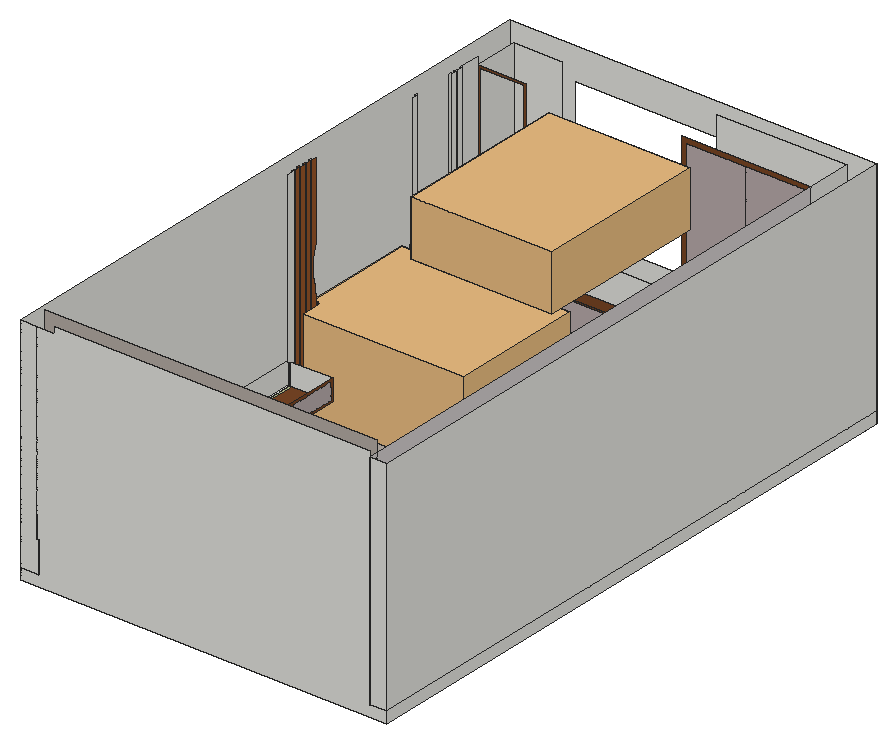
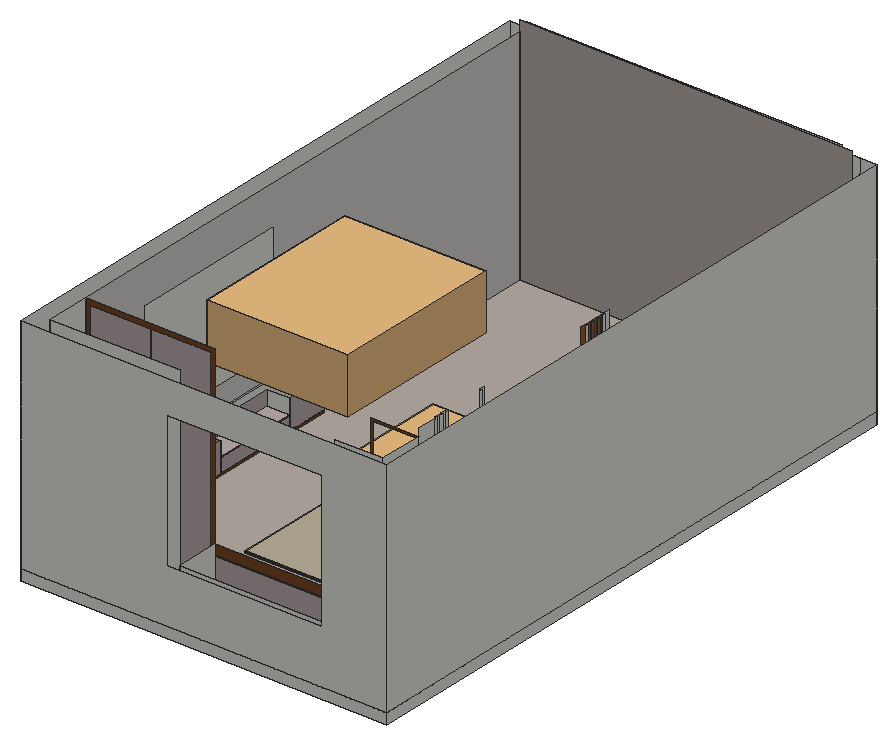
# SketchUp Ruby script. Lengths in inches.
U = 1.inch
M = Sketchup.active_model
def pt(a) = Geom::Point3d.new(a.map { |v| v * U })
def face(e, loops, mat)
  f = e.add_face(loops[0].map { |a| pt(a) })
  loops[1..].each { |l| e.add_face(l.map { |a| pt(a) }).erase! }
  f.material = f.back_material = mat if mat
  f
end
# faces: each face lists its corners as indices into pts; further lists are holes
def faces(e, pts, list, mat = nil) = list.each { |f| face(e, (f[0].is_a?(Array) ? f : [f]).map { |l| l.map { |i| pts[i] } }, mat) }
# xy, xz, yz: faces in a plane at the given z, y or x. An outline is a flat list of corners, or four numbers for a rectangle; further outlines are holes
def ring(l) = l.size == 4 ? [[l[0], l[1]], [l[2], l[1]], [l[2], l[3]], [l[0], l[3]]] : l.each_slice(2).to_a
def flat(e, list, mat, &to3) = list.each { |f| face(e, (f[0].is_a?(Array) ? f : [f]).map { |l| ring(l).map { |u, v| to3.(u, v) } }, mat) }
def xy(e, z, list, mat = nil) = flat(e, list, mat) { |x, y| [x, y, z] }
def xz(e, y, list, mat = nil) = flat(e, list, mat) { |x, z| [x, y, z] }
def yz(e, x, list, mat = nil) = flat(e, list, mat) { |y, z| [x, y, z] }
def lines(e, pts, list) = list.each { |a, b| e.add_line(pt(pts[a]), pt(pts[b])) }
# prism: a flat outline (further loops are holes) pulled along v
def prism(e, loops, v, mat = nil)
  f = face(e, loops, mat); d = Geom::Vector3d.new(v.map { |x| x * U })
  f.pushpull(f.normal.samedirection?(d) ? d.length : -d.length)
end
def box(e, o, s, mat = nil) = prism(e, [[o, [o[0] + s[0], o[1], o[2]], [o[0] + s[0], o[1] + s[1], o[2]], [o[0], o[1] + s[1], o[2]]]], [0, 0, s[2]], mat)
def at(x, y, z, deg = 0) = Geom::Transformation.translation(pt([x, y, z])) * Geom::Transformation.rotation(ORIGIN, Z_AXIS, deg.degrees)
def axes(o, x, y, z) = Geom::Transformation.new([*x, 0, *y, 0, *z, 0, *pt(o).to_a, 1])
def part(name) = M.definitions.add(name)
# library, detail: a bought-in or finely detailed component or shape, given as its bounding box
def library(name, o, s) = part(name).tap { |d| box(d.entities, o, s) }
def detail(e, o, s) = box(e.add_group.entities, o, s)
def put(e, d, t, mat = nil) = e.add_instance(d, t).tap { |i| i.material = mat if mat }
def group(e, t, mat = nil) = e.add_group.tap { |g| g.transformation = t; g.material = mat if mat }.entities
root = M.entities
M.materials.add("Ashlee 5_ x 8_").color = [182, 173, 150]
M.materials.add("Emissive").color = [188, 193, 143]
M.materials.add("Generic").color = [183, 170, 170]
M.materials.add("Generic\#1").color = [209, 204, 204]
M.materials.add("Tiles L01 200cm").color = [180, 171, 163]
M.materials.add("[Wood Cherry Original]").color = [152, 86, 42]
M.materials.add("[Wood Veneer 01]").color = [120, 70, 37]
c1 = library("ceiling fan",[0,0,0],[76.25,93.13,30.02])
c2 = part("fan")
p = [[217.527,-902.72,540.318],[217.529,-902.72,540.318],[217.529,-902.72,541.354],[217.527,-902.72,541.354]]
lines(c2.entities,p,[[0,1],[2,3]])
put(c2.entities,c1,at(256.45,-350.9,679.41))
c3 = library("BED 3",[-244.73,-59.6875,196.6875],[91.01,69.4,39.64])
c4 = part(" rug 5'x8'\#1")
xy(c4.entities,0,[[0,0,60,96]],"Ashlee 5_ x 8_")
xy(c4.entities,0.75,[[0.25,0.25,59.75,95.75]],"Ashlee 5_ x 8_")
xz(c4.entities,0,[[0,0,60,0.5]],"Ashlee 5_ x 8_")
xz(c4.entities,96,[[0,0,60,0.5]],"Ashlee 5_ x 8_")
yz(c4.entities,0,[[0,0,96,0.5]],"Ashlee 5_ x 8_")
yz(c4.entities,60,[[0,0,96,0.5]],"Ashlee 5_ x 8_")
p = [[59.99,0.01,0.56],[0.01,0.01,0.56],[0,0,0.5],[60,0,0.5],[0.01,95.99,0.56],[0,96,0.5],
  [59.99,95.99,0.56],[60,96,0.5],[0.03,0.03,0.625],[0.03,95.97,0.625],[59.97,0.03,0.625],[59.93,0.07,0.68],
  [0.07,0.07,0.68],[0.07,95.93,0.68],[59.93,95.93,0.68],[59.97,95.97,0.625],[0.125,0.125,0.72],[0.125,95.875,0.72],
  [59.81,0.19,0.74],[0.19,0.19,0.74],[59.875,0.125,0.72],[0.19,95.81,0.74],[59.81,95.81,0.74],[59.875,95.875,0.72],
  [0.25,0.25,0.75],[0.25,95.75,0.75],[59.75,0.25,0.75],[59.75,95.75,0.75]]
faces(c4.entities,p,[[0,1,2,3],[1,4,5,2],[6,0,3,7],[4,6,7,5],[8,9,4,1],[10,8,1,0],[11,12,8,10],[12,13,9,8],
  [14,11,10,15],[15,10,0,6],[13,14,15,9],[9,15,6,4],[16,17,13,12],[18,19,16,20],[20,16,12,11],[19,21,17,16],
  [22,18,20,23],[23,20,11,14],[24,25,21,19],[26,24,19,18],[27,26,18,22],[21,22,23,17],[25,27,22,21],[17,23,14,13]],"Ashlee 5_ x 8_")
xy(root,-6,[[0,0,198,331.1875]])
xy(root,0,[[0,0,9.9375,0,9.9375,172.18,9,172.18,9,173.55,9.9375,173.55,9.9375,175.97,9,175.97,9,177.34,9.9375,177.34,9.9375,179.77,9,179.77,9,181.13,9.9375,181.13,9.9375,183.56,9,183.56,9,184.92,9.9375,184.92,9.9375,187.35,9,187.35,9,188.71,9.8125,188.71,9.8125,191.14,9,191.14,9,192.51,9.8125,192.51,9.8125,194.93,9,194.93,9,196.3,9.8125,196.3,9.8125,198.72,9,198.72,9,200.09,9.8125,200.09,9.8125,202.52,9,202.52,9,203.88,9.8125,203.88,9.8125,206.31,9,206.31,9,207.67,9.8125,207.67,9.8125,210.1,9,210.1,9,211.46,9.8125,211.46,9.8125,213.89,9,213.89,9,215.26,9.8125,215.26,9.8125,217.68,9,217.68,9,219.05,9.8125,219.05,9.8125,221.47,9,221.47,9,222.84,9.8125,222.84,9.8125,225.27,9,225.27,9,226.63,9.8125,226.63,9.8125,229.06,9,229.06,9,230.42,9.8125,230.42,9.8125,232.85,9,232.85,9,234.21,9.8125,234.21,9.8125,236.64,9,236.64,9,238.01,9.8125,238.01,9.8125,240.43,9,240.43,9,241.8,9.8125,241.8,9.8125,244.22,9,244.22,9,245.59,9.8125,245.59,9.8125,248.02,9,248.02,9,249.38,9.8125,249.38,9.8125,251.81,9,251.81,9,253.17,9.8125,253.17,9.8125,255.6,9,255.6,9,279.71,9.8125,279.71,9.8125,282.14,9,282.14,9,283.51,9.8125,283.51,9.8125,285.93,9,285.93,9,322.1875,189,322.1875,189,0,198,0,198,331.1875,0,331.1875],[9,255.72,35,278.35],[9,298.1875,35,322.1875],[119,298.1875,189,322.1875],[35,302.1875,119,322.1875]])
xy(root,0,[[9.9375,5.08,189,5.08,189,298.1875,119,298.1875,119,302.1875,35,302.1875,35,298.1875,9,298.1875,9,285.93,9.8125,285.93,9.8125,283.51,9,283.51,9,282.14,9.8125,282.14,9.8125,279.71,9,279.71,9,278.35,35,278.35,35,255.72,9,255.72,9,255.6,9.8125,255.6,9.8125,253.17,9,253.17,9,251.81,9.8125,251.81,9.8125,249.38,9,249.38,9,248.02,9.8125,248.02,9.8125,245.59,9,245.59,9,244.22,9.8125,244.22,9.8125,241.8,9,241.8,9,240.43,9.8125,240.43,9.8125,238.01,9,238.01,9,236.64,9.8125,236.64,9.8125,234.21,9,234.21,9,232.85,9.8125,232.85,9.8125,230.42,9,230.42,9,229.06,9.8125,229.06,9.8125,226.63,9,226.63,9,225.27,9.8125,225.27,9.8125,222.84,9,222.84,9,221.47,9.8125,221.47,9.8125,219.05,9,219.05,9,217.68,9.8125,217.68,9.8125,215.26,9,215.26,9,213.89,9.8125,213.89,9.8125,211.46,9,211.46,9,210.1,9.8125,210.1,9.8125,207.67,9,207.67,9,206.31,9.8125,206.31,9.8125,203.88,9,203.88,9,202.52,9.8125,202.52,9.8125,200.09,9,200.09,9,198.72,9.8125,198.72,9.8125,196.3,9,196.3,9,194.93,9.8125,194.93,9.8125,192.51,9,192.51,9,191.14,9.8125,191.14,9.8125,188.71,9,188.71,9,187.35,9.9375,187.35,9.9375,184.92,9,184.92,9,183.56,9.9375,183.56,9.9375,181.13,9,181.13,9,179.77,9.9375,179.77,9.9375,177.34,9,177.34,9,175.97,9.9375,175.97,9.9375,173.55,9,173.55,9,172.18,9.9375,172.18]],"Tiles L01 200cm")
xy(root,4,[[9,298.1875,35,322.1875],[119,298.1875,189,322.1875]])
xy(root,4,[[35,301.1875,119,302.1875]],"Emissive")
xy(root,4,[[35,298.1875,119,301.1875]],"[Wood Veneer 01]")
xy(root,8.125,[[188,157.25,189,273.75]],"Emissive")
xy(root,8.125,[[173,157.25,188,273.75]],"[Wood Veneer 01]")
xy(root,9.125,[[173,157.25,189,273.75]])
xy(root,9.5,[[173,157.25,189,273.75]])
xy(root,17.375,[[9,5.08,9.9375,133.1875],[9,133.1875,9.9375,169.5625]])
xy(root,17.375,[[9.9375,133.1875,11.19,169.5625]],"Emissive")
xy(root,17.375,[[9,0,9.9375,5.08]],"Tiles L01 200cm")
xy(root,17.375,[[11.19,133.1875,33.125,169.5625]],"[Wood Veneer 01]")
xy(root,17.4375,[[173,180.55,185,227.15]],"Generic")
xz(root,0,[[0,-6,198,-6,198,0,189,0,189,123,18.5,123,18.5,120,9,120,9,17.375,9.9375,17.375,9.9375,0,0,0],[0,0,9.9375,0,9.9375,17.375,9,17.375,9,120,0,120],[189,0,198,120]])
xz(root,5.08,[[9.9375,0,9.9375,17.375,9,17.375,9,126,189,126,189,0]],"Tiles L01 200cm")
xz(root,133.1875,[[9,17.375,33.125,29]],"[Wood Veneer 01]")
xz(root,157.25,[[173,8.125,189,9.125],[173,9.125,189,9.5],[173,9.5,189,25.375]],"[Wood Veneer 01]")
xz(root,169.5625,[[9,17.375,9.9375,29],[9.9375,17.375,33.125,29]])
xz(root,172.18,[[9,0,9.9375,120]])
xz(root,173.55,[[9,0,9.9375,120]])
xz(root,175.97,[[9,0,9.9375,120]])
xz(root,177.34,[[9,0,9.9375,120]],"[Wood Cherry Original]")
xz(root,179.77,[[9,0,9.9375,120]])
xz(root,180.55,[[173,17.4375,185,25.375]])
xz(root,181.13,[[9,0,9.9375,120]],"[Wood Cherry Original]")
xz(root,183.56,[[9,0,9.9375,120]])
xz(root,184.92,[[9,0,9.9375,120]],"[Wood Cherry Original]")
xz(root,187.35,[[9,0,9.9375,52.97]])
xz(root,188.71,[[9,0,9.8125,49.35]])
xz(root,191.14,[[9,0,9.8125,45.43]])
xz(root,192.51,[[9,0,9.8125,43.75]])
xz(root,194.93,[[9,0,9.8125,41.75]])
xz(root,196.3,[[9,0,9.8125,41.75]])
xz(root,198.72,[[9,0,9.8125,41.75]])
xz(root,200.09,[[9,0,9.8125,41.75]])
xz(root,202.52,[[9,0,9.8125,41.75]])
xz(root,203.88,[[9,0,9.8125,41.75]])
xz(root,206.31,[[9,0,9.8125,41.75]])
xz(root,207.67,[[9,0,9.8125,41.75]])
xz(root,210.1,[[9,0,9.8125,41.75]])
xz(root,211.46,[[9,0,9.8125,41.75]])
xz(root,213.89,[[9,0,9.8125,41.75]])
xz(root,215.26,[[9,0,9.8125,41.75]])
xz(root,217.68,[[9,0,9.8125,41.75]])
xz(root,219.05,[[9,0,9.8125,41.75]])
xz(root,221.47,[[9,0,9.8125,41.75]])
xz(root,222.84,[[9,0,9.8125,41.75]])
xz(root,225.27,[[9,0,9.8125,41.75]])
xz(root,226.63,[[9,0,9.8125,41.75]])
xz(root,227.15,[[173,17.4375,185,25.375]],"Generic")
xz(root,229.06,[[9,0,9.8125,41.75]])
xz(root,230.42,[[9,0,9.8125,41.75]])
xz(root,232.85,[[9,0,9.8125,41.75]])
xz(root,234.21,[[9,0,9.8125,41.75]])
xz(root,236.64,[[9,0,9.8125,41.75]])
xz(root,238.01,[[9,0,9.8125,41.75]])
xz(root,240.43,[[9,0,9.8125,42.02]])
xz(root,241.8,[[9,0,9.8125,42.2]])
xz(root,244.22,[[9,0,9.8125,42.92]])
xz(root,245.59,[[9,0,9.8125,43.49]])
xz(root,248.02,[[9,0,9.8125,44.92]])
xz(root,249.38,[[9,0,9.8125,45.96]],"Emissive")
xz(root,251.81,[[9,0,9.8125,48.63]])
xz(root,253.17,[[9,0,9.8125,50.64]])
xz(root,255.6,[[9,0,9.8125,120]])
xz(root,255.72,[[9,0,35,20.75]],"[Wood Veneer 01]")
xz(root,273.75,[[173,8.125,189,9.125],[173,9.125,189,9.5],[173,9.5,189,25.375]])
xz(root,278.35,[[9,0,9,23.75,9.8125,23.75,9.8125,20.75,35,20.75,35,0]],"[Wood Veneer 01]")
xz(root,279.71,[[9,0,9.8125,120]])
xz(root,282.14,[[9,0,9.8125,120]])
xz(root,283.51,[[9,0,9.8125,120]])
xz(root,285.93,[[9,0,9.8125,120]])
xz(root,298.1875,[[35,4,119,19.375],[121.42,6.42,153.6,117.58],[154,6.42,186.58,117.58]],"Generic")
xz(root,298.1875,[[9,0,35,4],[119,0,189,4],[[9,4,35,116],[10,5,10,115,34,115,34,92,34.03,92,34.03,70,34,70,34,48,34.03,48,34.03,26,34,26,34,5]],[[119,4,189,120],[121.42,6.42,186.58,117.58]],[10,5,34,5,34,26,10.03,26,10.03,27,10,27],
  [153.6,6.42,154,117.58],[35,19.375,119,20.125],[35,20.125,119,25.25]],"[Wood Veneer 01]")
xz(root,302.1875,[[35,0,119,4]],"[Wood Veneer 01]")
xz(root,322.1875,[[9,0,35,4],[35,0,119,25.25],[119,0,189,4],[9,4,35,116],[119,4,189,120]])
xz(root,331.1875,[[0,-6,198,0],[[0,0,198,120],[35,29.13,119,102.58]]])
yz(root,0,[[0,-6,331.1875,0],[0,0,331.1875,120]])
yz(root,9,[[172.18,0,173.55,120],[183.56,0,184.92,120],[187.35,0,188.71,0,188.71,49.35,188.15,50.54,187.35,52.97],[191.14,0,192.51,0,192.51,43.75,192.41,43.92,191.14,45.43],[194.93,0,196.3,41.75],
  [198.72,0,200.09,41.75],[202.52,0,203.88,41.75],[206.31,0,207.67,41.75],[210.1,0,211.46,41.75],[213.89,0,215.26,41.75],
  [217.68,0,219.05,41.75],[221.47,0,222.84,41.75],[225.27,0,226.63,41.75],[229.06,0,230.42,41.75],[232.85,0,234.21,41.75],
  [236.64,0,238.01,41.75],[240.43,0,241.8,0,241.8,42.2,240.43,42.02],[244.22,0,245.59,0,245.59,43.49,244.22,42.92],[248.02,0,249.38,0,249.38,45.96,248.02,44.92],[251.81,0,253.17,0,253.17,50.64,252.97,50.14,251.81,48.63],
  [255.6,0,255.72,0,255.72,21.61,256.96,21.61,256.96,120,255.6,120],[255.72,0,256.96,20.75],[256.96,0,259.39,23.75],[259.39,0,260.76,20.75],[260.76,0,263.18,23.75],
  [263.18,0,264.55,20.75],[264.55,0,266.97,23.75],[266.97,0,268.34,20.75],[268.34,0,270.77,23.75],[270.77,0,272.13,20.75],
  [272.13,0,274.56,23.75],[274.56,0,275.92,20.75],[275.92,0,278.35,23.75],[278.35,0,279.71,120],[282.14,0,283.51,120],
  [285.93,0,287.3,120],[287.3,0,298.1875,120],[298.1875,0,322.1875,4],[298.1875,4,322.1875,116],[0,17.375,5.08,29],
  [5.08,17.375,133.1875,29],[133.1875,17.375,169.5625,29]])
yz(root,9,[[175.97,0,177.34,120],[179.77,0,181.13,120]],"[Wood Cherry Original]")
yz(root,9.8125,[[188.71,0,191.14,0,191.14,45.43,190.71,45.9375,189.28,48.16,188.71,49.35],[192.51,0,194.93,0,194.93,41.75,193.62,41.75,192.51,43.75],[196.3,0,198.72,41.75],[200.09,0,202.52,41.75],[203.88,0,206.31,41.75],
  [207.67,0,210.1,41.75],[211.46,0,213.89,41.75],[215.26,0,217.68,41.75],[219.05,0,221.47,41.75],[222.84,0,225.27,41.75],
  [226.63,0,229.06,41.75],[230.42,0,232.85,41.75],[234.21,0,236.64,41.75],[238.01,0,240.43,0,240.43,42.02,238.43,41.75,238.01,41.75],[241.8,0,244.22,0,244.22,42.92,242.78,42.32,241.8,42.2],
  [245.59,0,248.02,0,248.02,44.92,246.82,44,245.59,43.49],[249.38,0,251.81,0,251.81,48.63,250.3,46.67,249.38,45.96],[253.17,0,255.6,0,255.6,120,253.17,120,253.17,66.43,254.64,62.875,255.21,58.53,254.64,54.19,253.17,50.64],[279.71,0,282.14,120],[283.51,0,285.93,120]])
yz(root,9.9375,[[0,0,5.08,17.375],[5.08,0,172.18,0,172.18,120,168.67,120,168.67,29,169.5625,29,169.5625,17.375,5.08,17.375]])
yz(root,9.9375,[[173.55,0,175.97,120],[177.34,0,179.77,120],[181.13,0,183.56,120],[184.92,0,187.35,0,187.35,52.97,187.33,53.04,186.83,55.63,186.66,58.26,186,60.8125,185.55,63.41,185.32,66.03,185.31,68.66,185.51,71.29,185.9375,73.88,186.57,76.4375,187.35,78.74,187.35,120,184.92,120]],"[Wood Cherry Original]")
yz(root,33.125,[[134.55,18.74,168.2,27.64]],"Generic")
yz(root,33.125,[[[133.1875,17.375,169.5625,29],[134.55,18.74,168.2,27.64]]],"[Wood Veneer 01]")
yz(root,35,[[302.1875,0,322.1875,4],[298.1875,4,322.1875,25.25]])
yz(root,35,[[255.72,0,278.35,0,278.35,20.75,277.21,20.75,277.21,1.14,256.86,1.14,256.86,20.75,255.72,20.75],[298.1875,0,302.1875,4],[256.86,1.14,277.21,11.875],[256.86,11.875,277.21,12.28],[256.86,12.28,277.21,20.75]],"[Wood Veneer 01]")
yz(root,119,[[302.1875,0,322.1875,4],[298.1875,4,322.1875,25.25]])
yz(root,119,[[298.1875,0,302.1875,4]],"[Wood Veneer 01]")
yz(root,173,[[157.25,9.5,180.15,25.375],[180.55,9.5,227.15,17.04],[227.55,9.5,250.05,25.375],[250.45,9.5,273.75,25.375]],"Generic")
yz(root,173,[[157.25,8.125,273.75,9.125],[157.25,9.125,273.75,9.5],[180.15,9.5,180.55,25.375],[227.15,9.5,227.55,25.375],[250.05,9.5,250.45,25.375],
  [180.55,17.04,227.15,17.4375]],"[Wood Veneer 01]")
yz(root,185,[[180.55,17.4375,227.15,25.375]],"Generic")
yz(root,189,[[298.1875,0,322.1875,4],[298.1875,4,322.1875,120],[157.25,8.125,273.75,9.125],[157.25,9.125,273.75,9.5],[157.25,9.5,273.75,25.375]])
yz(root,189,[[0,0,5.08,120],[[5.08,0,298.1875,120],[170.86,38.02,259.23,99.15],[157.25,8.125,273.75,26.625]]],"Generic\#1")
yz(root,198,[[0,-6,331.1875,0],[0,0,331.1875,120]])
put(root,c2,at(-189.375,531.26,-585.29))
put(root,c3,axes([250.79,240.19,-242.45],[1,0,0],[0,1.03755,0],[0,0,1.23]))
put(root,c4,at(72.82,165.1,0))
